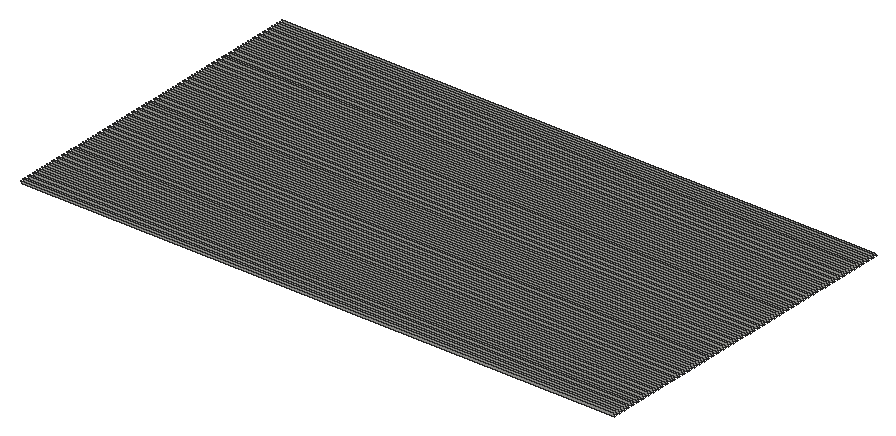
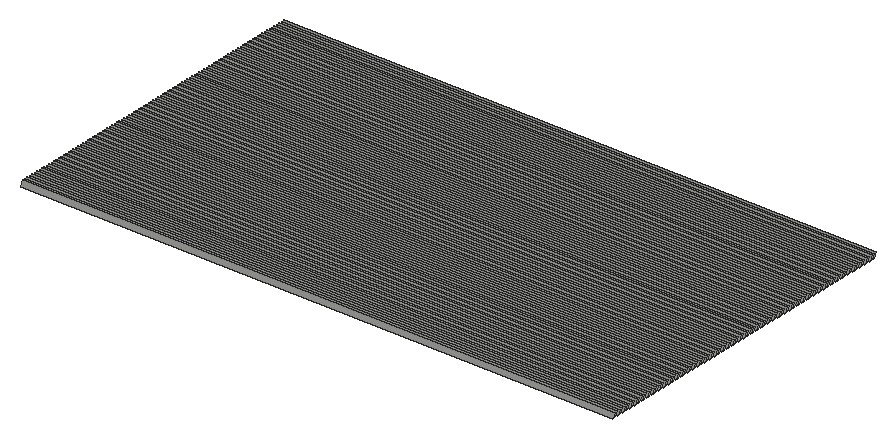
# SketchUp Ruby script. Lengths in inches.
U = 1.inch
M = Sketchup.active_model
def pt(a) = Geom::Point3d.new(a.map { |v| v * U })
def face(e, loops, mat)
  f = e.add_face(loops[0].map { |a| pt(a) })
  loops[1..].each { |l| e.add_face(l.map { |a| pt(a) }).erase! }
  f.material = f.back_material = mat if mat
  f
end
# faces: each face lists its corners as indices into pts; further lists are holes
def faces(e, pts, list, mat = nil) = list.each { |f| face(e, (f[0].is_a?(Array) ? f : [f]).map { |l| l.map { |i| pts[i] } }, mat) }
# xy, xz, yz: faces in a plane at the given z, y or x. An outline is a flat list of corners, or four numbers for a rectangle; further outlines are holes
def ring(l) = l.size == 4 ? [[l[0], l[1]], [l[2], l[1]], [l[2], l[3]], [l[0], l[3]]] : l.each_slice(2).to_a
def flat(e, list, mat, &to3) = list.each { |f| face(e, (f[0].is_a?(Array) ? f : [f]).map { |l| ring(l).map { |u, v| to3.(u, v) } }, mat) }
def xy(e, z, list, mat = nil) = flat(e, list, mat) { |x, y| [x, y, z] }
def xz(e, y, list, mat = nil) = flat(e, list, mat) { |x, z| [x, y, z] }
def yz(e, x, list, mat = nil) = flat(e, list, mat) { |y, z| [x, y, z] }
def lines(e, pts, list) = list.each { |a, b| e.add_line(pt(pts[a]), pt(pts[b])) }
# prism: a flat outline (further loops are holes) pulled along v
def prism(e, loops, v, mat = nil)
  f = face(e, loops, mat); d = Geom::Vector3d.new(v.map { |x| x * U })
  f.pushpull(f.normal.samedirection?(d) ? d.length : -d.length)
end
def box(e, o, s, mat = nil) = prism(e, [[o, [o[0] + s[0], o[1], o[2]], [o[0] + s[0], o[1] + s[1], o[2]], [o[0], o[1] + s[1], o[2]]]], [0, 0, s[2]], mat)
def at(x, y, z, deg = 0) = Geom::Transformation.translation(pt([x, y, z])) * Geom::Transformation.rotation(ORIGIN, Z_AXIS, deg.degrees)
def axes(o, x, y, z) = Geom::Transformation.new([*x, 0, *y, 0, *z, 0, *pt(o).to_a, 1])
def part(name) = M.definitions.add(name)
# library, detail: a bought-in or finely detailed component or shape, given as its bounding box
def library(name, o, s) = part(name).tap { |d| box(d.entities, o, s) }
def detail(e, o, s) = box(e.add_group.entities, o, s)
def put(e, d, t, mat = nil) = e.add_instance(d, t).tap { |i| i.material = mat if mat }
def group(e, t, mat = nil) = e.add_group.tap { |g| g.transformation = t; g.material = mat if mat }.entities
root = M.entities
c1 = part("Group209\#1")
p = [[385.16,-232.3,0],[-385.16,-232.3,0],[-385.16,-235.6875,5.875],[385.16,-235.6875,5.875]]
faces(c1.entities,p,[[0,1,2,3]])
c2 = part("Group210\#1")
p = [[385.16,-228.36,0],[-385.16,-228.36,0],[-385.16,-231.75,5.875],[385.16,-231.75,5.875]]
faces(c2.entities,p,[[0,1,2,3]])
c3 = part("Group211\#1")
p = [[-385.16,-227.8125,5.875],[385.16,-227.8125,5.875],[385.16,-224.42,0],[-385.16,-224.42,0]]
faces(c3.entities,p,[[0,1,2,3]])
c4 = part("Group212\#1")
p = [[-385.16,-223.875,5.875],[385.16,-223.875,5.875],[385.16,-220.48,0],[-385.16,-220.48,0]]
faces(c4.entities,p,[[0,1,2,3]])
c5 = part("Group213\#1")
p = [[-385.16,-219.9375,5.875],[385.16,-219.9375,5.875],[385.16,-216.55,0],[-385.16,-216.55,0]]
faces(c5.entities,p,[[0,1,2,3]])
c6 = part("Group214\#1")
p = [[385.16,-212.61,0],[-385.16,-212.61,0],[-385.16,-216,5.875],[385.16,-216,5.875]]
faces(c6.entities,p,[[0,1,2,3]])
c7 = part("Group215\#1")
p = [[385.16,-208.67,0],[-385.16,-208.67,0],[-385.16,-212.0625,5.875],[385.16,-212.0625,5.875]]
faces(c7.entities,p,[[0,1,2,3]])
c8 = part("Group216\#1")
p = [[385.16,-204.73,0],[-385.16,-204.73,0],[-385.16,-208.125,5.875],[385.16,-208.125,5.875]]
faces(c8.entities,p,[[0,1,2,3]])
c9 = part("Group217\#1")
p = [[385.16,-200.8,0],[-385.16,-200.8,0],[-385.16,-204.1875,5.875],[385.16,-204.1875,5.875]]
faces(c9.entities,p,[[0,1,2,3]])
c10 = part("Group218\#1")
p = [[385.16,-196.86,0],[-385.16,-196.86,0],[-385.16,-200.25,5.875],[385.16,-200.25,5.875]]
faces(c10.entities,p,[[0,1,2,3]])
c11 = part("Group219\#1")
p = [[385.16,-192.92,0],[-385.16,-192.92,0],[-385.16,-196.3125,5.875],[385.16,-196.3125,5.875]]
faces(c11.entities,p,[[0,1,2,3]])
c12 = part("Group220\#1")
p = [[-385.16,-192.375,5.875],[385.16,-192.375,5.875],[385.16,-188.98,0],[-385.16,-188.98,0]]
faces(c12.entities,p,[[0,1,2,3]])
c13 = part("Group221\#1")
p = [[385.16,-185.05,0],[-385.16,-185.05,0],[-385.16,-188.4375,5.875],[385.16,-188.4375,5.875]]
faces(c13.entities,p,[[0,1,2,3]])
c14 = part("Group222\#1")
p = [[385.16,-181.11,0],[-385.16,-181.11,0],[-385.16,-184.5,5.875],[385.16,-184.5,5.875]]
faces(c14.entities,p,[[0,1,2,3]])
c15 = part("Group223\#1")
p = [[-385.16,-180.5625,5.875],[385.16,-180.5625,5.875],[385.16,-177.17,0],[-385.16,-177.17,0]]
faces(c15.entities,p,[[0,1,2,3]])
c16 = part("Group224\#1")
p = [[385.16,-173.23,0],[-385.16,-173.23,0],[-385.16,-176.625,5.875],[385.16,-176.625,5.875]]
faces(c16.entities,p,[[0,1,2,3]])
c17 = part("Group225\#1")
p = [[-385.16,-172.6875,5.875],[385.16,-172.6875,5.875],[385.16,-169.3,0],[-385.16,-169.3,0]]
faces(c17.entities,p,[[0,1,2,3]])
c18 = part("Group226\#1")
p = [[-385.16,-168.75,5.875],[385.16,-168.75,5.875],[385.16,-165.36,0],[-385.16,-165.36,0]]
faces(c18.entities,p,[[0,1,2,3]])
c19 = part("Group227\#1")
p = [[-385.16,-164.8125,5.875],[385.16,-164.8125,5.875],[385.16,-161.42,0],[-385.16,-161.42,0]]
faces(c19.entities,p,[[0,1,2,3]])
c20 = part("Group228\#1")
p = [[-385.16,-160.875,5.875],[385.16,-160.875,5.875],[385.16,-157.48,0],[-385.16,-157.48,0]]
faces(c20.entities,p,[[0,1,2,3]])
c21 = part("Group229\#1")
p = [[-385.16,-156.9375,5.875],[385.16,-156.9375,5.875],[385.16,-153.55,0],[-385.16,-153.55,0]]
faces(c21.entities,p,[[0,1,2,3]])
c22 = part("Group230\#1")
p = [[385.16,-149.61,0],[-385.16,-149.61,0],[-385.16,-153,5.875],[385.16,-153,5.875]]
faces(c22.entities,p,[[0,1,2,3]])
c23 = part("Group231\#1")
p = [[-385.16,-149.0625,5.875],[385.16,-149.0625,5.875],[385.16,-145.67,0],[-385.16,-145.67,0]]
faces(c23.entities,p,[[0,1,2,3]])
c24 = part("Group232\#1")
p = [[385.16,-141.73,0],[-385.16,-141.73,0],[-385.16,-145.125,5.875],[385.16,-145.125,5.875]]
faces(c24.entities,p,[[0,1,2,3]])
c25 = part("Group233\#1")
p = [[-385.16,-141.1875,5.875],[385.16,-141.1875,5.875],[385.16,-137.8,0],[-385.16,-137.8,0]]
faces(c25.entities,p,[[0,1,2,3]])
c26 = part("Group234\#1")
p = [[385.16,-133.86,0],[-385.16,-133.86,0],[-385.16,-137.25,5.875],[385.16,-137.25,5.875]]
faces(c26.entities,p,[[0,1,2,3]])
c27 = part("Group235\#1")
p = [[-385.16,-133.3125,5.875],[385.16,-133.3125,5.875],[385.16,-129.92,0],[-385.16,-129.92,0]]
faces(c27.entities,p,[[0,1,2,3]])
c28 = part("Group236\#1")
p = [[-385.16,-129.375,5.875],[385.16,-129.375,5.875],[385.16,-125.98,0],[-385.16,-125.98,0]]
faces(c28.entities,p,[[0,1,2,3]])
c29 = part("Group237\#1")
p = [[385.16,-122.05,0],[-385.16,-122.05,0],[-385.16,-125.4375,5.875],[385.16,-125.4375,5.875]]
faces(c29.entities,p,[[0,1,2,3]])
c30 = part("Group238\#1")
p = [[-385.16,-121.5,5.875],[385.16,-121.5,5.875],[385.16,-118.11,0],[-385.16,-118.11,0]]
faces(c30.entities,p,[[0,1,2,3]])
c31 = part("Group239\#1")
p = [[385.16,-114.17,0],[-385.16,-114.17,0],[-385.16,-117.5625,5.875],[385.16,-117.5625,5.875]]
faces(c31.entities,p,[[0,1,2,3]])
c32 = part("Group240\#1")
p = [[385.16,-110.23,0],[-385.16,-110.23,0],[-385.16,-113.625,5.875],[385.16,-113.625,5.875]]
faces(c32.entities,p,[[0,1,2,3]])
c33 = part("Group241\#1")
p = [[385.16,-106.3,0],[-385.16,-106.3,0],[-385.16,-109.6875,5.875],[385.16,-109.6875,5.875]]
faces(c33.entities,p,[[0,1,2,3]])
c34 = part("Group242\#1")
p = [[-385.16,-105.75,5.875],[385.16,-105.75,5.875],[385.16,-102.36,0],[-385.16,-102.36,0]]
faces(c34.entities,p,[[0,1,2,3]])
c35 = part("Group243\#1")
p = [[385.16,-98.42,0],[-385.16,-98.42,0],[-385.16,-101.8125,5.875],[385.16,-101.8125,5.875]]
faces(c35.entities,p,[[0,1,2,3]])
c36 = part("Group244\#1")
p = [[385.16,-94.48,0],[-385.16,-94.48,0],[-385.16,-97.875,5.875],[385.16,-97.875,5.875]]
faces(c36.entities,p,[[0,1,2,3]])
c37 = part("Group245\#1")
p = [[-385.16,-93.9375,5.875],[385.16,-93.9375,5.875],[385.16,-90.55,0],[-385.16,-90.55,0]]
faces(c37.entities,p,[[0,1,2,3]])
c38 = part("Group246\#1")
p = [[385.16,-86.61,0],[-385.16,-86.61,0],[-385.16,-90,5.875],[385.16,-90,5.875]]
faces(c38.entities,p,[[0,1,2,3]])
c39 = part("Group247\#1")
p = [[-385.16,-86.0625,5.875],[385.16,-86.0625,5.875],[385.16,-82.67,0],[-385.16,-82.67,0]]
faces(c39.entities,p,[[0,1,2,3]])
c40 = part("Group248\#1")
p = [[385.16,-78.73,0],[-385.16,-78.73,0],[-385.16,-82.125,5.875],[385.16,-82.125,5.875]]
faces(c40.entities,p,[[0,1,2,3]])
c41 = part("Group249\#1")
p = [[-385.16,-78.1875,5.875],[385.16,-78.1875,5.875],[385.16,-74.8,0],[-385.16,-74.8,0]]
faces(c41.entities,p,[[0,1,2,3]])
c42 = part("Group250\#1")
p = [[385.16,-70.86,0],[-385.16,-70.86,0],[-385.16,-74.25,5.875],[385.16,-74.25,5.875]]
faces(c42.entities,p,[[0,1,2,3]])
c43 = part("Group251\#1")
p = [[-385.16,-70.3125,5.875],[385.16,-70.3125,5.875],[385.16,-66.92,0],[-385.16,-66.92,0]]
faces(c43.entities,p,[[0,1,2,3]])
c44 = part("Group252\#1")
p = [[385.16,-62.98,0],[-385.16,-62.98,0],[-385.16,-66.375,5.875],[385.16,-66.375,5.875]]
faces(c44.entities,p,[[0,1,2,3]])
c45 = part("Group253\#1")
p = [[-385.16,-62.4375,5.875],[385.16,-62.4375,5.875],[385.16,-59.05,0],[-385.16,-59.05,0]]
faces(c45.entities,p,[[0,1,2,3]])
c46 = part("Group254\#1")
p = [[-385.16,-58.5,5.875],[385.16,-58.5,5.875],[385.16,-55.11,0],[-385.16,-55.11,0]]
faces(c46.entities,p,[[0,1,2,3]])
c47 = part("Group255\#1")
p = [[-385.16,-54.5625,5.875],[385.16,-54.5625,5.875],[385.16,-51.17,0],[-385.16,-51.17,0]]
faces(c47.entities,p,[[0,1,2,3]])
c48 = part("Group256\#1")
p = [[385.16,-47.23,0],[-385.16,-47.23,0],[-385.16,-50.625,5.875],[385.16,-50.625,5.875]]
faces(c48.entities,p,[[0,1,2,3]])
c49 = part("Group257\#1")
p = [[-385.16,-46.6875,5.875],[385.16,-46.6875,5.875],[385.16,-43.3,0],[-385.16,-43.3,0]]
faces(c49.entities,p,[[0,1,2,3]])
c50 = part("Group258\#1")
p = [[385.16,-39.36,0],[-385.16,-39.36,0],[-385.16,-42.75,5.875],[385.16,-42.75,5.875]]
faces(c50.entities,p,[[0,1,2,3]])
c51 = part("Group259\#1")
p = [[-385.16,-38.8125,5.875],[385.16,-38.8125,5.875],[385.16,-35.42,0],[-385.16,-35.42,0]]
faces(c51.entities,p,[[0,1,2,3]])
c52 = part("Group260\#1")
p = [[385.16,-31.48,0],[-385.16,-31.48,0],[-385.16,-34.875,5.875],[385.16,-34.875,5.875]]
faces(c52.entities,p,[[0,1,2,3]])
c53 = part("Group261\#1")
p = [[-385.16,-30.9375,5.875],[385.16,-30.9375,5.875],[385.16,-27.55,0],[-385.16,-27.55,0]]
faces(c53.entities,p,[[0,1,2,3]])
c54 = part("Group262\#1")
p = [[385.16,-23.61,0],[-385.16,-23.61,0],[-385.16,-27,5.875],[385.16,-27,5.875]]
faces(c54.entities,p,[[0,1,2,3]])
c55 = part("Group263\#1")
p = [[-385.16,-23.0625,5.875],[385.16,-23.0625,5.875],[385.16,-19.67,0],[-385.16,-19.67,0]]
faces(c55.entities,p,[[0,1,2,3]])
c56 = part("Group264\#1")
p = [[385.16,-15.73,0],[-385.16,-15.73,0],[-385.16,-19.125,5.875],[385.16,-19.125,5.875]]
faces(c56.entities,p,[[0,1,2,3]])
c57 = part("Group265\#1")
p = [[385.16,-11.8,0],[-385.16,-11.8,0],[-385.16,-15.1875,5.875],[385.16,-15.1875,5.875]]
faces(c57.entities,p,[[0,1,2,3]])
c58 = part("Group266\#1")
p = [[385.16,-7.86,0],[-385.16,-7.86,0],[-385.16,-11.25,5.875],[385.16,-11.25,5.875]]
faces(c58.entities,p,[[0,1,2,3]])
c59 = part("Group267\#1")
p = [[385.16,-3.92,0],[-385.16,-3.92,0],[-385.16,-7.3125,5.875],[385.16,-7.3125,5.875]]
faces(c59.entities,p,[[0,1,2,3]])
c60 = part("Group268\#1")
p = [[-385.16,-3.375,5.875],[385.16,-3.375,5.875],[385.16,0.02,0],[-385.16,0.02,0]]
faces(c60.entities,p,[[0,1,2,3]])
c61 = part("Group269\#1")
p = [[-385.16,0.5625,5.875],[385.16,0.5625,5.875],[385.16,3.95,0],[-385.16,3.95,0]]
faces(c61.entities,p,[[0,1,2,3]])
c62 = part("Group270\#1")
p = [[-385.16,4.5,5.875],[385.16,4.5,5.875],[385.16,7.89,0],[-385.16,7.89,0]]
faces(c62.entities,p,[[0,1,2,3]])
c63 = part("Group271\#1")
p = [[-385.16,8.4375,5.875],[385.16,8.4375,5.875],[385.16,11.83,0],[-385.16,11.83,0]]
faces(c63.entities,p,[[0,1,2,3]])
c64 = part("Group272\#1")
p = [[-385.16,12.375,5.875],[385.16,12.375,5.875],[385.16,15.77,0],[-385.16,15.77,0]]
faces(c64.entities,p,[[0,1,2,3]])
c65 = part("Group273\#1")
p = [[-385.16,16.3125,5.875],[385.16,16.3125,5.875],[385.16,19.7,0],[-385.16,19.7,0]]
faces(c65.entities,p,[[0,1,2,3]])
c66 = part("Group274\#1")
p = [[-385.16,20.25,5.875],[385.16,20.25,5.875],[385.16,23.64,0],[-385.16,23.64,0]]
faces(c66.entities,p,[[0,1,2,3]])
c67 = part("Group275\#1")
p = [[385.16,27.58,0],[-385.16,27.58,0],[-385.16,24.1875,5.875],[385.16,24.1875,5.875]]
faces(c67.entities,p,[[0,1,2,3]])
c68 = part("Group276\#1")
p = [[-385.16,28.125,5.875],[385.16,28.125,5.875],[385.16,31.52,0],[-385.16,31.52,0]]
faces(c68.entities,p,[[0,1,2,3]])
c69 = part("Group277\#1")
p = [[-385.16,32.0625,5.875],[385.16,32.0625,5.875],[385.16,35.45,0],[-385.16,35.45,0]]
faces(c69.entities,p,[[0,1,2,3]])
c70 = part("Group278\#1")
p = [[385.16,39.39,0],[-385.16,39.39,0],[-385.16,36,5.875],[385.16,36,5.875]]
faces(c70.entities,p,[[0,1,2,3]])
c71 = part("Group279\#1")
p = [[385.16,43.33,0],[-385.16,43.33,0],[-385.16,39.9375,5.875],[385.16,39.9375,5.875]]
faces(c71.entities,p,[[0,1,2,3]])
c72 = part("Group280\#1")
p = [[385.16,47.27,0],[-385.16,47.27,0],[-385.16,43.875,5.875],[385.16,43.875,5.875]]
faces(c72.entities,p,[[0,1,2,3]])
c73 = part("Group281\#1")
p = [[-385.16,47.8125,5.875],[385.16,47.8125,5.875],[385.16,51.2,0],[-385.16,51.2,0]]
faces(c73.entities,p,[[0,1,2,3]])
c74 = part("Group282\#1")
p = [[-385.16,51.75,5.875],[385.16,51.75,5.875],[385.16,55.14,0],[-385.16,55.14,0]]
faces(c74.entities,p,[[0,1,2,3]])
c75 = part("Group283\#1")
p = [[-385.16,55.6875,5.875],[385.16,55.6875,5.875],[385.16,59.08,0],[-385.16,59.08,0]]
faces(c75.entities,p,[[0,1,2,3]])
c76 = part("Group284\#1")
p = [[-385.16,59.625,5.875],[385.16,59.625,5.875],[385.16,63.02,0],[-385.16,63.02,0]]
faces(c76.entities,p,[[0,1,2,3]])
c77 = part("Group285\#1")
p = [[-385.16,63.5625,5.875],[385.16,63.5625,5.875],[385.16,66.95,0],[-385.16,66.95,0]]
faces(c77.entities,p,[[0,1,2,3]])
c78 = part("Group286\#1")
p = [[385.16,70.89,0],[-385.16,70.89,0],[-385.16,67.5,5.875],[385.16,67.5,5.875]]
faces(c78.entities,p,[[0,1,2,3]])
c79 = part("Group287\#1")
p = [[385.16,74.83,0],[-385.16,74.83,0],[-385.16,71.4375,5.875],[385.16,71.4375,5.875]]
faces(c79.entities,p,[[0,1,2,3]])
c80 = part("Group288\#1")
p = [[-385.16,75.375,5.875],[385.16,75.375,5.875],[385.16,78.77,0],[-385.16,78.77,0]]
faces(c80.entities,p,[[0,1,2,3]])
c81 = part("Group289\#1")
p = [[385.16,82.7,0],[-385.16,82.7,0],[-385.16,79.3125,5.875],[385.16,79.3125,5.875]]
faces(c81.entities,p,[[0,1,2,3]])
c82 = part("Group290\#1")
p = [[-385.16,83.25,5.875],[385.16,83.25,5.875],[385.16,86.64,0],[-385.16,86.64,0]]
faces(c82.entities,p,[[0,1,2,3]])
c83 = part("Group291\#1")
p = [[-385.16,87.1875,5.875],[385.16,87.1875,5.875],[385.16,90.58,0],[-385.16,90.58,0]]
faces(c83.entities,p,[[0,1,2,3]])
c84 = part("Group292\#1")
p = [[-385.16,91.125,5.875],[385.16,91.125,5.875],[385.16,94.52,0],[-385.16,94.52,0]]
faces(c84.entities,p,[[0,1,2,3]])
c85 = part("Group293\#1")
p = [[385.16,98.45,0],[-385.16,98.45,0],[-385.16,95.0625,5.875],[385.16,95.0625,5.875]]
faces(c85.entities,p,[[0,1,2,3]])
c86 = part("Group294\#1")
p = [[385.16,102.39,0],[-385.16,102.39,0],[-385.16,99,5.875],[385.16,99,5.875]]
faces(c86.entities,p,[[0,1,2,3]])
c87 = part("Group295\#1")
p = [[-385.16,102.9375,5.875],[385.16,102.9375,5.875],[385.16,106.33,0],[-385.16,106.33,0]]
faces(c87.entities,p,[[0,1,2,3]])
c88 = part("Group296\#1")
p = [[385.16,110.27,0],[-385.16,110.27,0],[-385.16,106.875,5.875],[385.16,106.875,5.875]]
faces(c88.entities,p,[[0,1,2,3]])
c89 = part("Group297\#1")
p = [[-385.16,110.8125,5.875],[385.16,110.8125,5.875],[385.16,114.2,0],[-385.16,114.2,0]]
faces(c89.entities,p,[[0,1,2,3]])
c90 = part("Group298\#1")
p = [[385.16,118.14,0],[-385.16,118.14,0],[-385.16,114.75,5.875],[385.16,114.75,5.875]]
faces(c90.entities,p,[[0,1,2,3]])
c91 = part("Group299\#1")
p = [[385.16,122.08,0],[-385.16,122.08,0],[-385.16,118.6875,5.875],[385.16,118.6875,5.875]]
faces(c91.entities,p,[[0,1,2,3]])
c92 = part("Group300\#1")
p = [[-385.16,122.625,5.875],[385.16,122.625,5.875],[385.16,126.02,0],[-385.16,126.02,0]]
faces(c92.entities,p,[[0,1,2,3]])
c93 = part("Group301\#1")
p = [[-385.16,126.5625,5.875],[385.16,126.5625,5.875],[385.16,129.95,0],[-385.16,129.95,0]]
faces(c93.entities,p,[[0,1,2,3]])
c94 = part("Group302\#1")
p = [[385.16,133.89,0],[-385.16,133.89,0],[-385.16,130.5,5.875],[385.16,130.5,5.875]]
faces(c94.entities,p,[[0,1,2,3]])
c95 = part("Group303\#1")
p = [[385.16,137.83,0],[-385.16,137.83,0],[-385.16,134.4375,5.875],[385.16,134.4375,5.875]]
faces(c95.entities,p,[[0,1,2,3]])
c96 = part("Group304\#1")
p = [[-385.16,138.375,5.875],[385.16,138.375,5.875],[385.16,141.77,0],[-385.16,141.77,0]]
faces(c96.entities,p,[[0,1,2,3]])
c97 = part("Group305\#1")
p = [[385.16,145.7,0],[-385.16,145.7,0],[-385.16,142.3125,5.875],[385.16,142.3125,5.875]]
faces(c97.entities,p,[[0,1,2,3]])
c98 = part("Group306\#1")
p = [[-385.16,146.25,5.875],[385.16,146.25,5.875],[385.16,149.64,0],[-385.16,149.64,0]]
faces(c98.entities,p,[[0,1,2,3]])
c99 = part("Group307\#1")
p = [[-385.16,150.1875,5.875],[385.16,150.1875,5.875],[385.16,153.58,0],[-385.16,153.58,0]]
faces(c99.entities,p,[[0,1,2,3]])
c100 = part("Group308\#1")
p = [[-385.16,154.125,5.875],[385.16,154.125,5.875],[385.16,157.52,0],[-385.16,157.52,0]]
faces(c100.entities,p,[[0,1,2,3]])
c101 = part("Group309\#1")
p = [[-385.16,158.0625,5.875],[385.16,158.0625,5.875],[385.16,161.45,0],[-385.16,161.45,0]]
faces(c101.entities,p,[[0,1,2,3]])
c102 = part("Group310\#1")
p = [[-385.16,162,5.875],[385.16,162,5.875],[385.16,165.39,0],[-385.16,165.39,0]]
faces(c102.entities,p,[[0,1,2,3]])
c103 = part("Group311\#1")
p = [[-385.16,165.9375,5.875],[385.16,165.9375,5.875],[385.16,169.33,0],[-385.16,169.33,0]]
faces(c103.entities,p,[[0,1,2,3]])
c104 = part("Group312\#1")
p = [[-385.16,169.875,5.875],[385.16,169.875,5.875],[385.16,173.27,0],[-385.16,173.27,0]]
faces(c104.entities,p,[[0,1,2,3]])
c105 = part("Group313\#1")
p = [[-385.16,173.8125,5.875],[385.16,173.8125,5.875],[385.16,177.2,0],[-385.16,177.2,0]]
faces(c105.entities,p,[[0,1,2,3]])
c106 = part("Group314\#1")
p = [[385.16,181.14,0],[-385.16,181.14,0],[-385.16,177.75,5.875],[385.16,177.75,5.875]]
faces(c106.entities,p,[[0,1,2,3]])
c107 = part("Group315\#1")
p = [[-385.16,181.6875,5.875],[385.16,181.6875,5.875],[385.16,185.08,0],[-385.16,185.08,0]]
faces(c107.entities,p,[[0,1,2,3]])
c108 = part("Group316\#1")
p = [[-385.16,185.625,5.875],[385.16,185.625,5.875],[385.16,189.02,0],[-385.16,189.02,0]]
faces(c108.entities,p,[[0,1,2,3]])
c109 = part("Group317\#1")
p = [[385.16,192.95,0],[-385.16,192.95,0],[-385.16,189.5625,5.875],[385.16,189.5625,5.875]]
faces(c109.entities,p,[[0,1,2,3]])
put(root,c1,at(1937.93,1232.46,154.625))
put(root,c2,at(1937.93,1232.46,154.625))
put(root,c3,at(1937.93,1232.46,154.625))
put(root,c4,at(1937.93,1232.46,154.625))
put(root,c5,at(1937.93,1232.46,154.625))
put(root,c6,at(1937.93,1232.46,154.625))
put(root,c7,at(1937.93,1232.46,154.625))
put(root,c8,at(1937.93,1232.46,154.625))
put(root,c9,at(1937.93,1232.46,154.625))
put(root,c10,at(1937.93,1232.46,154.625))
put(root,c11,at(1937.93,1232.46,154.625))
put(root,c12,at(1937.93,1232.46,154.625))
put(root,c13,at(1937.93,1232.46,154.625))
put(root,c14,at(1937.93,1232.46,154.625))
put(root,c15,at(1937.93,1232.46,154.625))
put(root,c16,at(1937.93,1232.46,154.625))
put(root,c17,at(1937.93,1232.46,154.625))
put(root,c18,at(1937.93,1232.46,154.625))
put(root,c19,at(1937.93,1232.46,154.625))
put(root,c20,at(1937.93,1232.46,154.625))
put(root,c21,at(1937.93,1232.46,154.625))
put(root,c22,at(1937.93,1232.46,154.625))
put(root,c23,at(1937.93,1232.46,154.625))
put(root,c24,at(1937.93,1232.46,154.625))
put(root,c25,at(1937.93,1232.46,154.625))
put(root,c26,at(1937.93,1232.46,154.625))
put(root,c27,at(1937.93,1232.46,154.625))
put(root,c28,at(1937.93,1232.46,154.625))
put(root,c29,at(1937.93,1232.46,154.625))
put(root,c30,at(1937.93,1232.46,154.625))
put(root,c31,at(1937.93,1232.46,154.625))
put(root,c32,at(1937.93,1232.46,154.625))
put(root,c33,at(1937.93,1232.46,154.625))
put(root,c34,at(1937.93,1232.46,154.625))
put(root,c35,at(1937.93,1232.46,154.625))
put(root,c36,at(1937.93,1232.46,154.625))
put(root,c37,at(1937.93,1232.46,154.625))
put(root,c38,at(1937.93,1232.46,154.625))
put(root,c39,at(1937.93,1232.46,154.625))
put(root,c40,at(1937.93,1232.46,154.625))
put(root,c41,at(1937.93,1232.46,154.625))
put(root,c42,at(1937.93,1232.46,154.625))
put(root,c43,at(1937.93,1232.46,154.625))
put(root,c44,at(1937.93,1232.46,154.625))
put(root,c45,at(1937.93,1232.46,154.625))
put(root,c46,at(1937.93,1232.46,154.625))
put(root,c47,at(1937.93,1232.46,154.625))
put(root,c48,at(1937.93,1232.46,154.625))
put(root,c49,at(1937.93,1232.46,154.625))
put(root,c50,at(1937.93,1232.46,154.625))
put(root,c51,at(1937.93,1232.46,154.625))
put(root,c52,at(1937.93,1232.46,154.625))
put(root,c53,at(1937.93,1232.46,154.625))
put(root,c54,at(1937.93,1232.46,154.625))
put(root,c55,at(1937.93,1232.46,154.625))
put(root,c56,at(1937.93,1232.46,154.625))
put(root,c57,at(1937.93,1232.46,154.625))
put(root,c58,at(1937.93,1232.46,154.625))
put(root,c59,at(1937.93,1232.46,154.625))
put(root,c60,at(1937.93,1232.46,154.625))
put(root,c61,at(1937.93,1232.46,154.625))
put(root,c62,at(1937.93,1232.46,154.625))
put(root,c63,at(1937.93,1232.46,154.625))
put(root,c64,at(1937.93,1232.46,154.625))
put(root,c65,at(1937.93,1232.46,154.625))
put(root,c66,at(1937.93,1232.46,154.625))
put(root,c67,at(1937.93,1232.46,154.625))
put(root,c68,at(1937.93,1232.46,154.625))
put(root,c69,at(1937.93,1232.46,154.625))
put(root,c70,at(1937.93,1232.46,154.625))
put(root,c71,at(1937.93,1232.46,154.625))
put(root,c72,at(1937.93,1232.46,154.625))
put(root,c73,at(1937.93,1232.46,154.625))
put(root,c74,at(1937.93,1232.46,154.625))
put(root,c75,at(1937.93,1232.46,154.625))
put(root,c76,at(1937.93,1232.46,154.625))
put(root,c77,at(1937.93,1232.46,154.625))
put(root,c78,at(1937.93,1232.46,154.625))
put(root,c79,at(1937.93,1232.46,154.625))
put(root,c80,at(1937.93,1232.46,154.625))
put(root,c81,at(1937.93,1232.46,154.625))
put(root,c82,at(1937.93,1232.46,154.625))
put(root,c83,at(1937.93,1232.46,154.625))
put(root,c84,at(1937.93,1232.46,154.625))
put(root,c85,at(1937.93,1232.46,154.625))
put(root,c86,at(1937.93,1232.46,154.625))
put(root,c87,at(1937.93,1232.46,154.625))
put(root,c88,at(1937.93,1232.46,154.625))
put(root,c89,at(1937.93,1232.46,154.625))
put(root,c90,at(1937.93,1232.46,154.625))
put(root,c91,at(1937.93,1232.46,154.625))
put(root,c92,at(1937.93,1232.46,154.625))
put(root,c93,at(1937.93,1232.46,154.625))
put(root,c94,at(1937.93,1232.46,154.625))
put(root,c95,at(1937.93,1232.46,154.625))
put(root,c96,at(1937.93,1232.46,154.625))
put(root,c97,at(1937.93,1232.46,154.625))
put(root,c98,at(1937.93,1232.46,154.625))
put(root,c99,at(1937.93,1232.46,154.625))
put(root,c100,at(1937.93,1232.46,154.625))
put(root,c101,at(1937.93,1232.46,154.625))
put(root,c102,at(1937.93,1232.46,154.625))
put(root,c103,at(1937.93,1232.46,154.625))
put(root,c104,at(1937.93,1232.46,154.625))
put(root,c105,at(1937.93,1232.46,154.625))
put(root,c106,at(1937.93,1232.46,154.625))
put(root,c107,at(1937.93,1232.46,154.625))
put(root,c108,at(1937.93,1232.46,154.625))
put(root,c109,at(1937.93,1232.46,154.625))
